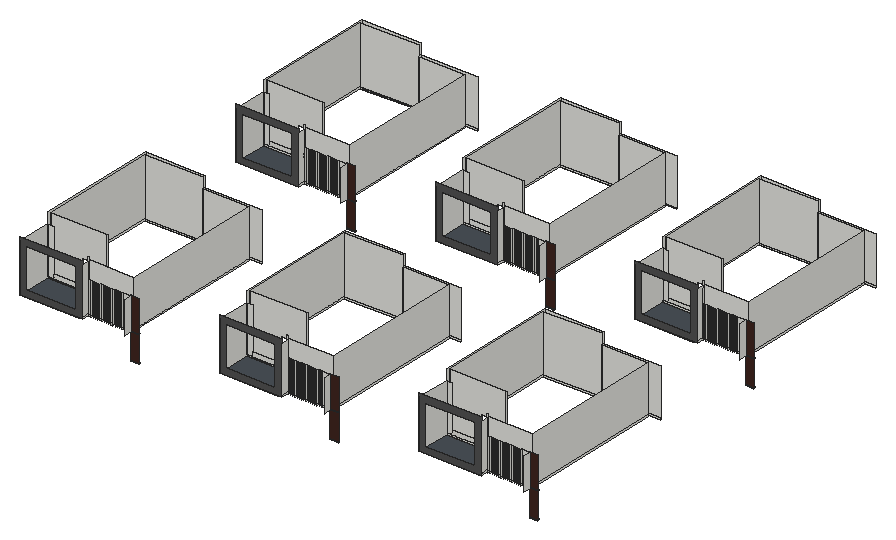
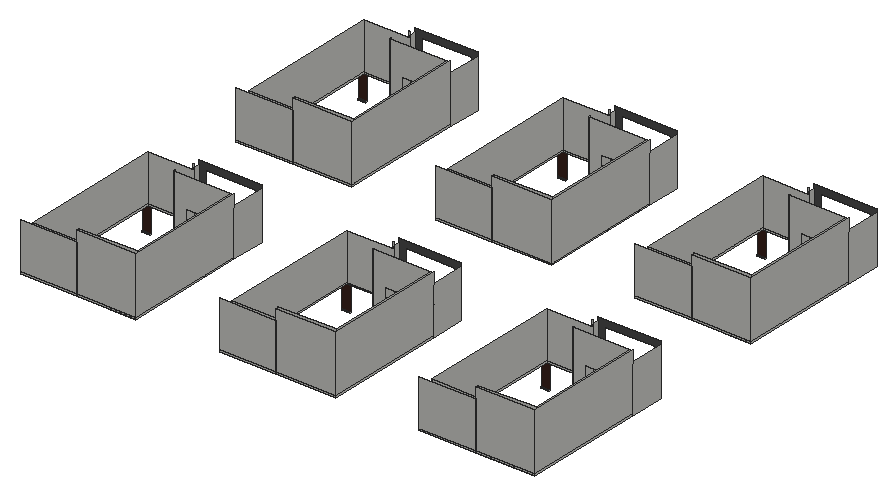
# SketchUp Ruby script. Lengths in inches.
U = 1.inch
M = Sketchup.active_model
def pt(a) = Geom::Point3d.new(a.map { |v| v * U })
def face(e, loops, mat)
  f = e.add_face(loops[0].map { |a| pt(a) })
  loops[1..].each { |l| e.add_face(l.map { |a| pt(a) }).erase! }
  f.material = f.back_material = mat if mat
  f
end
# faces: each face lists its corners as indices into pts; further lists are holes
def faces(e, pts, list, mat = nil) = list.each { |f| face(e, (f[0].is_a?(Array) ? f : [f]).map { |l| l.map { |i| pts[i] } }, mat) }
# xy, xz, yz: faces in a plane at the given z, y or x. An outline is a flat list of corners, or four numbers for a rectangle; further outlines are holes
def ring(l) = l.size == 4 ? [[l[0], l[1]], [l[2], l[1]], [l[2], l[3]], [l[0], l[3]]] : l.each_slice(2).to_a
def flat(e, list, mat, &to3) = list.each { |f| face(e, (f[0].is_a?(Array) ? f : [f]).map { |l| ring(l).map { |u, v| to3.(u, v) } }, mat) }
def xy(e, z, list, mat = nil) = flat(e, list, mat) { |x, y| [x, y, z] }
def xz(e, y, list, mat = nil) = flat(e, list, mat) { |x, z| [x, y, z] }
def yz(e, x, list, mat = nil) = flat(e, list, mat) { |y, z| [x, y, z] }
def lines(e, pts, list) = list.each { |a, b| e.add_line(pt(pts[a]), pt(pts[b])) }
# prism: a flat outline (further loops are holes) pulled along v
def prism(e, loops, v, mat = nil)
  f = face(e, loops, mat); d = Geom::Vector3d.new(v.map { |x| x * U })
  f.pushpull(f.normal.samedirection?(d) ? d.length : -d.length)
end
def box(e, o, s, mat = nil) = prism(e, [[o, [o[0] + s[0], o[1], o[2]], [o[0] + s[0], o[1] + s[1], o[2]], [o[0], o[1] + s[1], o[2]]]], [0, 0, s[2]], mat)
def at(x, y, z, deg = 0) = Geom::Transformation.translation(pt([x, y, z])) * Geom::Transformation.rotation(ORIGIN, Z_AXIS, deg.degrees)
def axes(o, x, y, z) = Geom::Transformation.new([*x, 0, *y, 0, *z, 0, *pt(o).to_a, 1])
def part(name) = M.definitions.add(name)
# library, detail: a bought-in or finely detailed component or shape, given as its bounding box
def library(name, o, s) = part(name).tap { |d| box(d.entities, o, s) }
def detail(e, o, s) = box(e.add_group.entities, o, s)
def put(e, d, t, mat = nil) = e.add_instance(d, t).tap { |i| i.material = mat if mat }
def group(e, t, mat = nil) = e.add_group.tap { |g| g.transformation = t; g.material = mat if mat }.entities
root = M.entities
M.materials.add("Glass_Tinted_Gray").color = [0, 0, 0]
M.materials["Glass_Tinted_Gray"].alpha = 0.125
M.materials.add("[0043_SaddleBrown]").color = [63, 38, 31]
M.materials.add("[0135_DarkGray]").color = [81, 81, 81]
M.materials.add("[Formica Blue]").color = [73, 80, 86]
M.materials.add("[Mirror 02]").color = [229, 229, 229]
M.materials.add("[Terrazzo Light Blue]").color = [196, 214, 227]
c1 = part("PENTEK_RP Fineline 50S_Sliding_DoorCase_E1")
box(c1.entities,[0,0,0],[1.51,3.66,99.27],"[0135_DarkGray]")
c2 = part("PENTEK_RP Fineline 50S_SlidingDooe_Case_E2")
box(c2.entities,[0,0,0],[96.25,3.66,1.51],"[0135_DarkGray]")
c3 = part("pentek_RP Fineline 50S_SlidingDoor_Case")
put(c3.entities,c1,at(97.76,0,0))
put(c3.entities,c2,at(1.51,0,0))
put(c3.entities,c1,at(0,0,0))
put(c3.entities,c2,at(1.51,0,97.76))
c4 = part("PENTEK_RP Fineline 50S_SlidingDoor_GlazingBead_2")
box(c4.entities,[0,0,0],[0.56,0.59,94.39],"[0135_DarkGray]")
c5 = part("PENTEK_RP Fineline 50S_SlidingDoor_Glass")
box(c5.entities,[0,0,0],[46.58,0.16,94.39],"Glass_Tinted_Gray")
c6 = part("PENTEK_RP Fineline 50S_SlidingDoor_GlazingBead")
box(c6.entities,[0,0,0],[45.47,0.59,0.56],"[0135_DarkGray]")
c7 = part("PENTEK_RP Fineline 50S_SlidingDoor_Leaf_E1")
xy(c7.entities,0,[[0,0,0.93,1.97],[0.93,1.57,1.49,1.97]],"[0135_DarkGray]")
xy(c7.entities,96.25,[[0,0,0.93,0,0.93,1.57,1.49,1.57,1.49,1.97,0,1.97]],"[0135_DarkGray]")
xz(c7.entities,0,[[0,0,0.93,96.25]],"[0135_DarkGray]")
xz(c7.entities,1.57,[[0.93,0,1.49,95.32],[0.93,95.32,1.49,96.25]],"[0135_DarkGray]")
xz(c7.entities,1.97,[[0,0,1.49,96.25]],"[0135_DarkGray]")
yz(c7.entities,0,[[0,0,1.97,96.25]],"[0135_DarkGray]")
yz(c7.entities,0.93,[[0,0,1.57,0.93],[0,0.93,1.57,95.32],[0,95.32,1.57,96.25]],"[0135_DarkGray]")
yz(c7.entities,1.49,[[1.57,0,1.97,95.32],[1.57,95.32,1.97,96.25]],"[0135_DarkGray]")
c8 = part("PENTEK_RP Fineline 50S_SlidingDoor_Leaf_E2")
xy(c8.entities,0,[[0,0,0,1.57,0.56,1.57,0.56,1.97,46.02,1.97,46.02,1.57,46.58,1.57,46.58,0]],"[0135_DarkGray]")
xy(c8.entities,0.93,[[0,0,46.58,1.57]],"[0135_DarkGray]")
xy(c8.entities,1.49,[[0.56,1.57,46.02,1.97]],"[0135_DarkGray]")
xz(c8.entities,0,[[0,0,46.58,0.93]],"[0135_DarkGray]")
xz(c8.entities,1.57,[[0,0,0.56,0.93],[46.02,0,46.58,0.93],[0.56,0.93,46.02,1.49]],"[0135_DarkGray]")
xz(c8.entities,1.97,[[0.56,0,46.02,1.49]],"[0135_DarkGray]")
yz(c8.entities,0,[[0,0,1.57,0.93]],"[0135_DarkGray]")
yz(c8.entities,0.56,[[1.57,0,1.97,0.93],[1.57,0.93,1.97,1.49]],"[0135_DarkGray]")
yz(c8.entities,46.02,[[1.57,0,1.97,0.93],[1.57,0.93,1.97,1.49]],"[0135_DarkGray]")
yz(c8.entities,46.58,[[0,0,1.57,0.93]],"[0135_DarkGray]")
c9 = part("PENTEK_RP Fineline S_SlidingDoor_Leaf1")
put(c9.entities,c4,at(0.93,0,0.93))
put(c9.entities,c4,at(46.96,0,0.93))
put(c9.entities,c5,at(1.49,1.42,0.93))
put(c9.entities,c6,at(1.49,0,0.93))
put(c9.entities,c5,at(1.49,0.59,0.93),"[Terrazzo Light Blue]")
put(c9.entities,c7,at(0,0,0))
put(c9.entities,c7,axes([48.44,0,0],[-1,0,0],[0,1,0],[0,0,1]))
put(c9.entities,c8,axes([0.93,0,96.25],[1,0,0],[0,1,0],[0,0,-1]))
put(c9.entities,c8,at(0.93,0,0))
put(c9.entities,c6,at(1.49,0,94.77))
c10 = part("PENTEK_RP Fineline 50S_SlidingDoor_Leaf2")
put(c10.entities,c5,at(1.49,1.42,0.93))
put(c10.entities,c6,at(1.49,0,94.77))
put(c10.entities,c4,at(46.96,0,0.93))
put(c10.entities,c5,at(1.49,0.59,0.93),"[Mirror 02]")
put(c10.entities,c4,at(0.93,0,0.93))
put(c10.entities,c7,at(0,0,0))
put(c10.entities,c7,axes([48.44,0,0],[-1,0,0],[0,1,0],[0,0,1]))
put(c10.entities,c6,at(1.49,0,0.93))
put(c10.entities,c8,axes([0.93,0,96.25],[1,0,0],[0,1,0],[0,0,-1]))
put(c10.entities,c8,at(0.93,0,0))
c11 = part("PENTEK - Slimmest Steel Sliding Door / Window\#1")
put(c11.entities,c3,at(0,-1.88,-0.09))
put(c11.entities,c9,at(1.51,-2.27,1.42))
put(c11.entities,c10,at(49.32,-0.3,1.42))
xy(root,409.48,[[517.3125,438.73,547.05,442.66],[1241.75,438.73,1271.49,442.66],[1966.1875,438.73,1995.93,442.66],[517.3125,1419.08,547.05,1423.01],[1241.75,1419.08,1271.49,1423.01],
  [1966.1875,1419.08,1995.93,1423.01]])
xy(root,412.48,[[517.3125,438.72,517.3125,442.66,547.05,442.66,547.05,438.73],[1241.75,438.72,1241.75,442.66,1271.49,442.66,1271.49,438.73],[1966.1875,438.72,1966.1875,442.66,1995.93,442.66,1995.93,438.73],[517.3125,1419.07,517.3125,1423.01,547.05,1423.01,547.05,1419.08],[1241.75,1419.07,1241.75,1423.01,1271.49,1423.01,1271.49,1419.08],
  [1966.1875,1419.07,1966.1875,1423.01,1995.93,1423.01,1995.93,1419.08]],"[0043_SaddleBrown]")
xy(root,441.5,[[258.09,535.375,309.84,598.8125],[982.53,535.375,1034.28,598.8125],[1706.96,535.375,1758.71,598.8125],[258.09,1515.73,309.84,1579.16],[982.53,1515.73,1034.28,1579.16],
  [1706.96,1515.73,1758.71,1579.16]])
xy(root,485.6875,[[183.3,535.375,231.3,598.8125],[258.09,535.375,309.84,598.8125],[907.74,535.375,955.74,598.8125],[982.53,535.375,1034.28,598.8125],[1632.17,535.375,1680.17,598.8125],
  [1706.96,535.375,1758.71,598.8125],[183.3,1515.73,231.3,1579.16],[258.09,1515.73,309.84,1579.16],[907.74,1515.73,955.74,1579.16],[982.53,1515.73,1034.28,1579.16],
  [1632.17,1515.73,1680.17,1579.16],[1706.96,1515.73,1758.71,1579.16]])
xy(root,504.25,[[348.1875,412.04,348.1875,437.1,352.41,437.1,352.41,438.72,353.97,438.72,353.97,412.04],[353.97,412.04,353.97,437.1,358.875,437.1,358.875,438.72,361.3,438.72,361.3,437.1,363.73,437.1,363.73,412.04],[1072.625,412.04,1072.625,437.1,1076.85,437.1,1076.85,438.72,1078.41,438.72,1078.41,412.04],[1078.41,412.04,1078.41,437.1,1083.3125,437.1,1083.3125,438.72,1085.74,438.72,1085.74,437.1,1088.17,437.1,1088.17,412.04],[1797.0625,412.04,1797.0625,437.1,1801.29,437.1,1801.29,438.72,1802.84,438.72,1802.84,412.04],
  [1802.84,412.04,1802.84,437.1,1807.75,437.1,1807.75,438.72,1810.18,438.72,1810.18,437.1,1812.6,437.1,1812.6,412.04],[348.1875,437.1,348.1875,447.84,353.97,447.84,353.97,438.72,352.41,438.72,352.41,437.1],[361.3,437.1,363.73,438.72],[1072.625,437.1,1072.625,447.84,1078.41,447.84,1078.41,438.72,1076.85,438.72,1076.85,437.1],[1085.74,437.1,1088.17,438.72],
  [1797.0625,437.1,1797.0625,447.84,1802.84,447.84,1802.84,438.72,1801.29,438.72,1801.29,437.1],[1810.18,437.1,1812.6,438.72],[137.5,535.375,137.5,980.35,353.97,980.35,353.97,971.23,144.84,965.96,144.84,540.48,353.97,540.48,353.97,535.375],[861.9375,535.375,861.9375,980.35,1078.41,980.35,1078.41,971.23,869.28,965.96,869.28,540.48,1078.41,540.48,1078.41,535.375],[1586.375,535.375,1586.375,980.35,1802.84,980.35,1802.84,971.23,1593.72,965.96,1593.72,540.48,1802.84,540.48,1802.84,535.375],
  [144.84,540.48,353.97,598.8125],[869.28,540.48,1078.41,598.8125],[1593.72,540.48,1802.84,598.8125],[348.1875,1392.39,348.1875,1417.45,352.41,1417.45,352.41,1419.07,353.97,1419.07,353.97,1392.39],[353.97,1392.39,353.97,1417.45,358.875,1417.45,358.875,1419.07,361.3,1419.07,361.3,1417.45,363.73,1417.45,363.73,1392.39],
  [1072.625,1392.39,1072.625,1417.45,1076.85,1417.45,1076.85,1419.07,1078.41,1419.07,1078.41,1392.39],[1078.41,1392.39,1078.41,1417.45,1083.3125,1417.45,1083.3125,1419.07,1085.74,1419.07,1085.74,1417.45,1088.17,1417.45,1088.17,1392.39],[1797.0625,1392.39,1797.0625,1417.45,1801.29,1417.45,1801.29,1419.07,1802.84,1419.07,1802.84,1392.39],[1802.84,1392.39,1802.84,1417.45,1807.75,1417.45,1807.75,1419.07,1810.18,1419.07,1810.18,1417.45,1812.6,1417.45,1812.6,1392.39],[348.1875,1417.45,348.1875,1428.19,353.97,1428.19,353.97,1419.07,352.41,1419.07,352.41,1417.45],
  [361.3,1417.45,363.73,1419.07],[1072.625,1417.45,1072.625,1428.19,1078.41,1428.19,1078.41,1419.07,1076.85,1419.07,1076.85,1417.45],[1085.74,1417.45,1088.17,1419.07],[1797.0625,1417.45,1797.0625,1428.19,1802.84,1428.19,1802.84,1419.07,1801.29,1419.07,1801.29,1417.45],[1810.18,1417.45,1812.6,1419.07],
  [137.5,1515.73,137.5,1960.7,353.97,1960.7,353.97,1951.58,144.84,1946.3125,144.84,1520.83,353.97,1520.83,353.97,1515.73],[861.9375,1515.73,861.9375,1960.7,1078.41,1960.7,1078.41,1951.58,869.28,1946.3125,869.28,1520.83,1078.41,1520.83,1078.41,1515.73],[1586.375,1515.73,1586.375,1960.7,1802.84,1960.7,1802.84,1951.58,1593.72,1946.3125,1593.72,1520.83,1802.84,1520.83,1802.84,1515.73],[144.84,1520.83,353.97,1579.16],[869.28,1520.83,1078.41,1579.16],
  [1593.72,1520.83,1802.84,1579.16]])
xy(root,504.25,[[137.5,412.04,137.5,535.375,353.97,535.375,353.97,447.84,348.1875,447.84,348.1875,412.04],[861.9375,412.04,861.9375,535.375,1078.41,535.375,1078.41,447.84,1072.625,447.84,1072.625,412.04],[1586.375,412.04,1586.375,535.375,1802.84,535.375,1802.84,447.84,1797.0625,447.84,1797.0625,412.04],[137.5,1392.39,137.5,1515.73,353.97,1515.73,353.97,1428.19,348.1875,1428.19,348.1875,1392.39],[861.9375,1392.39,861.9375,1515.73,1078.41,1515.73,1078.41,1428.19,1072.625,1428.19,1072.625,1392.39],
  [1586.375,1392.39,1586.375,1515.73,1802.84,1515.73,1802.84,1428.19,1797.0625,1428.19,1797.0625,1392.39]],"[Formica Blue]")
xy(root,505.6875,[[517.3125,438.73,547.05,442.66],[1241.75,438.73,1271.49,442.66],[1966.1875,438.73,1995.93,442.66],[517.3125,1419.08,547.05,1423.01],[1241.75,1419.08,1271.49,1423.01],
  [1966.1875,1419.08,1995.93,1423.01]])
xy(root,508.42,[[517.3125,438.72,517.3125,442.66,547.05,442.66,547.05,438.73],[1241.75,438.72,1241.75,442.66,1271.49,442.66,1271.49,438.73],[1966.1875,438.72,1966.1875,442.66,1995.93,442.66,1995.93,438.73],[517.3125,1419.07,517.3125,1423.01,547.05,1423.01,547.05,1419.08],[1241.75,1419.07,1241.75,1423.01,1271.49,1423.01,1271.49,1419.08],
  [1966.1875,1419.07,1966.1875,1423.01,1995.93,1423.01,1995.93,1419.08]])
xy(root,510.25,[[137.5,535.375,137.5,980.35,353.97,980.35,353.97,971.23,144.84,965.96,144.84,540.48,353.97,540.48,353.97,535.375],[861.9375,535.375,861.9375,980.35,1078.41,980.35,1078.41,971.23,869.28,965.96,869.28,540.48,1078.41,540.48,1078.41,535.375],[1586.375,535.375,1586.375,980.35,1802.84,980.35,1802.84,971.23,1593.72,965.96,1593.72,540.48,1802.84,540.48,1802.84,535.375],[137.5,1515.73,137.5,1960.7,353.97,1960.7,353.97,1951.58,144.84,1946.3125,144.84,1520.83,353.97,1520.83,353.97,1515.73],[861.9375,1515.73,861.9375,1960.7,1078.41,1960.7,1078.41,1951.58,869.28,1946.3125,869.28,1520.83,1078.41,1520.83,1078.41,1515.73],
  [1586.375,1515.73,1586.375,1960.7,1802.84,1960.7,1802.84,1951.58,1593.72,1946.3125,1593.72,1520.83,1802.84,1520.83,1802.84,1515.73]])
xz(root,412.04,[[[137.5,504.25,363.73,693.65],[158.83,526.75,338.6875,669.8125]],[[861.9375,504.25,1088.17,693.65],[883.27,526.75,1063.125,669.8125]],[[1586.375,504.25,1812.6,693.65],[1607.71,526.75,1787.5625,669.8125]]],"[0135_DarkGray]")
xz(root,438.72,[[361.3,504.25,363.73,693.65],[1085.74,504.25,1088.17,693.65],[1810.18,504.25,1812.6,693.65],[487.0625,510.25,517.3125,620.875],[1211.5,510.25,1241.75,620.875],
  [1935.9375,510.25,1966.1875,620.875]])
xz(root,442.66,[[517.3125,409.48,547.05,412.48],[1241.75,409.48,1271.49,412.48],[1966.1875,409.48,1995.93,412.48],[517.3125,505.6875,547.05,508.42],[1241.75,505.6875,1271.49,508.42],
  [1966.1875,505.6875,1995.93,508.42]],"[0043_SaddleBrown]")
xz(root,447.84,[[348.1875,504.25,353.97,526.75],[353.97,504.25,521.63,510.25],[1072.625,504.25,1078.41,526.75],[1078.41,504.25,1246.07,510.25],[1797.0625,504.25,1802.84,526.75],
  [1802.84,504.25,1970.51,510.25],[353.97,510.25,521.63,679.3125],[1078.41,510.25,1246.07,679.3125],[1802.84,510.25,1970.51,679.3125]])
xz(root,535.375,[[137.5,504.25,353.97,510.25],[861.9375,504.25,1078.41,510.25],[1586.375,504.25,1802.84,510.25],[137.5,510.25,158.83,679.3125],[158.83,510.25,353.97,526.75],
  [861.9375,510.25,883.27,679.3125],[883.27,510.25,1078.41,526.75],[1586.375,510.25,1607.71,679.3125],[1607.71,510.25,1802.84,526.75]])
xz(root,540.48,[[144.84,504.25,353.97,510.25],[869.28,504.25,1078.41,510.25],[1593.72,504.25,1802.84,510.25],[[144.84,510.25,353.97,718],[258.09,566.5625,309.84,610.75]],[[869.28,510.25,1078.41,718],[982.53,566.5625,1034.28,610.75]],
  [[1593.72,510.25,1802.84,718],[1706.96,566.5625,1758.71,610.75]]])
xz(root,598.8125,[[258.09,441.5,309.84,485.6875],[982.53,441.5,1034.28,485.6875],[1706.96,441.5,1758.71,485.6875]])
xz(root,971.23,[[353.97,504.25,521.63,510.25],[1078.41,504.25,1246.07,510.25],[1802.84,504.25,1970.51,510.25],[353.97,510.25,521.63,679.3125],[1078.41,510.25,1246.07,679.3125],
  [1802.84,510.25,1970.51,679.3125]])
xz(root,980.35,[[137.5,504.25,353.97,510.25],[353.97,504.25,558.625,510.25],[861.9375,504.25,1078.41,510.25],[1078.41,504.25,1283.0625,510.25],[1586.375,504.25,1802.84,510.25],
  [1802.84,504.25,2007.5,510.25],[137.5,510.25,353.97,718],[353.97,510.25,558.625,679.3125],[861.9375,510.25,1078.41,718],[1078.41,510.25,1283.0625,679.3125],
  [1586.375,510.25,1802.84,718],[1802.84,510.25,2007.5,679.3125]])
xz(root,1392.39,[[[137.5,504.25,363.73,693.65],[158.83,526.75,338.6875,669.8125]],[[861.9375,504.25,1088.17,693.65],[883.27,526.75,1063.125,669.8125]],[[1586.375,504.25,1812.6,693.65],[1607.71,526.75,1787.5625,669.8125]]],"[0135_DarkGray]")
xz(root,1419.07,[[361.3,504.25,363.73,693.65],[1085.74,504.25,1088.17,693.65],[1810.18,504.25,1812.6,693.65],[487.0625,510.25,517.3125,620.875],[1211.5,510.25,1241.75,620.875],
  [1935.9375,510.25,1966.1875,620.875]])
xz(root,1423.01,[[517.3125,409.48,547.05,412.48],[1241.75,409.48,1271.49,412.48],[1966.1875,409.48,1995.93,412.48],[517.3125,505.6875,547.05,508.42],[1241.75,505.6875,1271.49,508.42],
  [1966.1875,505.6875,1995.93,508.42]],"[0043_SaddleBrown]")
xz(root,1428.19,[[348.1875,504.25,353.97,526.75],[353.97,504.25,521.63,510.25],[1072.625,504.25,1078.41,526.75],[1078.41,504.25,1246.07,510.25],[1797.0625,504.25,1802.84,526.75],
  [1802.84,504.25,1970.51,510.25],[353.97,510.25,521.63,679.3125],[1078.41,510.25,1246.07,679.3125],[1802.84,510.25,1970.51,679.3125]])
xz(root,1515.73,[[137.5,504.25,353.97,510.25],[861.9375,504.25,1078.41,510.25],[1586.375,504.25,1802.84,510.25],[137.5,510.25,158.83,679.3125],[158.83,510.25,353.97,526.75],
  [861.9375,510.25,883.27,679.3125],[883.27,510.25,1078.41,526.75],[1586.375,510.25,1607.71,679.3125],[1607.71,510.25,1802.84,526.75]])
xz(root,1520.83,[[144.84,504.25,353.97,510.25],[869.28,504.25,1078.41,510.25],[1593.72,504.25,1802.84,510.25],[[144.84,510.25,353.97,718],[258.09,566.5625,309.84,610.75]],[[869.28,510.25,1078.41,718],[982.53,566.5625,1034.28,610.75]],
  [[1593.72,510.25,1802.84,718],[1706.96,566.5625,1758.71,610.75]]])
xz(root,1579.16,[[258.09,441.5,309.84,485.6875],[982.53,441.5,1034.28,485.6875],[1706.96,441.5,1758.71,485.6875]])
xz(root,1951.58,[[353.97,504.25,521.63,510.25],[1078.41,504.25,1246.07,510.25],[1802.84,504.25,1970.51,510.25],[353.97,510.25,521.63,679.3125],[1078.41,510.25,1246.07,679.3125],
  [1802.84,510.25,1970.51,679.3125]])
xz(root,1960.7,[[137.5,504.25,353.97,510.25],[353.97,504.25,558.625,510.25],[861.9375,504.25,1078.41,510.25],[1078.41,504.25,1283.0625,510.25],[1586.375,504.25,1802.84,510.25],
  [1802.84,504.25,2007.5,510.25],[137.5,510.25,353.97,718],[353.97,510.25,558.625,679.3125],[861.9375,510.25,1078.41,718],[1078.41,510.25,1283.0625,679.3125],
  [1586.375,510.25,1802.84,718],[1802.84,510.25,2007.5,679.3125]])
yz(root,137.5,[[412.04,504.25,535.375,679.3125],[535.375,504.25,980.35,510.25],[1392.39,504.25,1515.73,679.3125],[1515.73,504.25,1960.7,510.25],[535.375,510.25,980.35,718],
  [1515.73,510.25,1960.7,718]])
yz(root,144.84,[[540.48,504.25,965.96,510.25],[1520.83,504.25,1946.3125,510.25],[540.48,510.25,965.96,718],[1520.83,510.25,1946.3125,718]])
yz(root,258.09,[[535.375,441.5,598.8125,485.6875],[1515.73,441.5,1579.16,485.6875]])
yz(root,309.84,[[535.375,441.5,598.8125,485.6875],[1515.73,441.5,1579.16,485.6875]])
yz(root,353.97,[[447.84,504.25,535.375,526.75],[535.375,504.25,540.48,510.25],[971.23,504.25,980.35,510.25],[1428.19,504.25,1515.73,526.75],[1515.73,504.25,1520.83,510.25],
  [1951.58,504.25,1960.7,510.25],[535.375,510.25,540.48,718],[971.23,510.25,980.35,679.3125],[1515.73,510.25,1520.83,718],[1951.58,510.25,1960.7,679.3125]])
yz(root,363.73,[[412.04,504.25,437.1,510.25],[437.1,504.25,438.72,510.25],[1392.39,504.25,1417.45,510.25],[1417.45,504.25,1419.07,510.25],[412.04,510.25,437.1,679.3125],
  [437.1,510.25,438.72,679.3125],[1392.39,510.25,1417.45,679.3125],[1417.45,510.25,1419.07,679.3125]])
yz(root,367.0625,[[437.1,504.25,438.72,510.25],[1417.45,504.25,1419.07,510.25],[437.1,510.25,438.72,620.875],[1417.45,510.25,1419.07,620.875]])
yz(root,375.0625,[[437.1,504.25,438.72,510.25],[1417.45,504.25,1419.07,510.25],[437.1,510.25,438.72,620.875],[1417.45,510.25,1419.07,620.875]])
yz(root,383.0625,[[437.1,504.25,438.72,510.25],[1417.45,504.25,1419.07,510.25],[437.1,510.25,438.72,620.875],[1417.45,510.25,1419.07,620.875]])
yz(root,391.0625,[[437.1,504.25,438.72,510.25],[1417.45,504.25,1419.07,510.25],[437.1,510.25,438.72,620.875],[1417.45,510.25,1419.07,620.875]])
yz(root,399.0625,[[437.1,504.25,438.72,510.25],[1417.45,504.25,1419.07,510.25],[437.1,510.25,438.72,620.875],[1417.45,510.25,1419.07,620.875]])
yz(root,407.0625,[[437.1,504.25,438.72,510.25],[1417.45,504.25,1419.07,510.25],[437.1,510.25,438.72,620.875],[1417.45,510.25,1419.07,620.875]])
yz(root,415.0625,[[437.1,504.25,438.72,510.25],[1417.45,504.25,1419.07,510.25],[437.1,510.25,438.72,620.875],[1417.45,510.25,1419.07,620.875]])
yz(root,423.0625,[[437.1,504.25,438.72,510.25],[1417.45,504.25,1419.07,510.25],[437.1,510.25,438.72,620.875],[1417.45,510.25,1419.07,620.875]])
yz(root,431.0625,[[437.1,504.25,438.72,510.25],[1417.45,504.25,1419.07,510.25],[437.1,510.25,438.72,620.875],[1417.45,510.25,1419.07,620.875]])
yz(root,439.0625,[[437.1,504.25,438.72,510.25],[1417.45,504.25,1419.07,510.25],[437.1,510.25,438.72,620.875],[1417.45,510.25,1419.07,620.875]])
yz(root,447.0625,[[437.1,504.25,438.72,510.25],[1417.45,504.25,1419.07,510.25],[437.1,510.25,438.72,620.875],[1417.45,510.25,1419.07,620.875]])
yz(root,455.0625,[[437.1,504.25,438.72,510.25],[1417.45,504.25,1419.07,510.25],[437.1,510.25,438.72,620.875],[1417.45,510.25,1419.07,620.875]])
yz(root,463.0625,[[437.1,504.25,438.72,510.25],[1417.45,504.25,1419.07,510.25],[437.1,510.25,438.72,620.875],[1417.45,510.25,1419.07,620.875]])
yz(root,471.0625,[[437.1,504.25,438.72,510.25],[1417.45,504.25,1419.07,510.25],[437.1,510.25,438.72,620.875],[1417.45,510.25,1419.07,620.875]])
yz(root,479.0625,[[437.1,504.25,438.72,510.25],[1417.45,504.25,1419.07,510.25],[437.1,510.25,438.72,620.875],[1417.45,510.25,1419.07,620.875]])
yz(root,487.0625,[[437.1,504.25,438.72,510.25],[1417.45,504.25,1419.07,510.25],[437.1,510.25,438.72,620.875],[1417.45,510.25,1419.07,620.875]])
yz(root,517.3125,[[438.73,409.48,442.66,409.48,442.66,412.48,438.72,412.48],[1419.08,409.48,1423.01,409.48,1423.01,412.48,1419.07,412.48],[412.04,504.25,438.72,504.25,438.73,505.6875,438.72,508.42,438.72,620.875,412.04,620.875],[1392.39,504.25,1419.07,504.25,1419.08,505.6875,1419.07,508.42,1419.07,620.875,1392.39,620.875],[438.73,505.6875,442.66,505.6875,442.66,508.42,438.72,508.42],
  [1419.08,505.6875,1423.01,505.6875,1423.01,508.42,1419.07,508.42]])
yz(root,521.63,[[447.84,504.25,971.23,510.25],[1428.19,504.25,1951.58,510.25],[447.84,510.25,971.23,679.3125],[1428.19,510.25,1951.58,679.3125]])
yz(root,861.9375,[[412.04,504.25,535.375,679.3125],[535.375,504.25,980.35,510.25],[1392.39,504.25,1515.73,679.3125],[1515.73,504.25,1960.7,510.25],[535.375,510.25,980.35,718],
  [1515.73,510.25,1960.7,718]])
yz(root,869.28,[[540.48,504.25,965.96,510.25],[1520.83,504.25,1946.3125,510.25],[540.48,510.25,965.96,718],[1520.83,510.25,1946.3125,718]])
yz(root,982.53,[[535.375,441.5,598.8125,485.6875],[1515.73,441.5,1579.16,485.6875]])
yz(root,1034.28,[[535.375,441.5,598.8125,485.6875],[1515.73,441.5,1579.16,485.6875]])
yz(root,1078.41,[[447.84,504.25,535.375,526.75],[535.375,504.25,540.48,510.25],[971.23,504.25,980.35,510.25],[1428.19,504.25,1515.73,526.75],[1515.73,504.25,1520.83,510.25],
  [1951.58,504.25,1960.7,510.25],[535.375,510.25,540.48,718],[971.23,510.25,980.35,679.3125],[1515.73,510.25,1520.83,718],[1951.58,510.25,1960.7,679.3125]])
yz(root,1088.17,[[412.04,504.25,437.1,510.25],[437.1,504.25,438.72,510.25],[1392.39,504.25,1417.45,510.25],[1417.45,504.25,1419.07,510.25],[412.04,510.25,437.1,679.3125],
  [437.1,510.25,438.72,679.3125],[1392.39,510.25,1417.45,679.3125],[1417.45,510.25,1419.07,679.3125]])
yz(root,1091.5,[[437.1,504.25,438.72,510.25],[1417.45,504.25,1419.07,510.25],[437.1,510.25,438.72,620.875],[1417.45,510.25,1419.07,620.875]])
yz(root,1099.5,[[437.1,504.25,438.72,510.25],[1417.45,504.25,1419.07,510.25],[437.1,510.25,438.72,620.875],[1417.45,510.25,1419.07,620.875]])
yz(root,1107.5,[[437.1,504.25,438.72,510.25],[1417.45,504.25,1419.07,510.25],[437.1,510.25,438.72,620.875],[1417.45,510.25,1419.07,620.875]])
yz(root,1115.5,[[437.1,504.25,438.72,510.25],[1417.45,504.25,1419.07,510.25],[437.1,510.25,438.72,620.875],[1417.45,510.25,1419.07,620.875]])
yz(root,1123.5,[[437.1,504.25,438.72,510.25],[1417.45,504.25,1419.07,510.25],[437.1,510.25,438.72,620.875],[1417.45,510.25,1419.07,620.875]])
yz(root,1131.5,[[437.1,504.25,438.72,510.25],[1417.45,504.25,1419.07,510.25],[437.1,510.25,438.72,620.875],[1417.45,510.25,1419.07,620.875]])
yz(root,1139.5,[[437.1,504.25,438.72,510.25],[1417.45,504.25,1419.07,510.25],[437.1,510.25,438.72,620.875],[1417.45,510.25,1419.07,620.875]])
yz(root,1147.5,[[437.1,504.25,438.72,510.25],[1417.45,504.25,1419.07,510.25],[437.1,510.25,438.72,620.875],[1417.45,510.25,1419.07,620.875]])
yz(root,1155.5,[[437.1,504.25,438.72,510.25],[1417.45,504.25,1419.07,510.25],[437.1,510.25,438.72,620.875],[1417.45,510.25,1419.07,620.875]])
yz(root,1163.5,[[437.1,504.25,438.72,510.25],[1417.45,504.25,1419.07,510.25],[437.1,510.25,438.72,620.875],[1417.45,510.25,1419.07,620.875]])
yz(root,1171.5,[[437.1,504.25,438.72,510.25],[1417.45,504.25,1419.07,510.25],[437.1,510.25,438.72,620.875],[1417.45,510.25,1419.07,620.875]])
yz(root,1179.5,[[437.1,504.25,438.72,510.25],[1417.45,504.25,1419.07,510.25],[437.1,510.25,438.72,620.875],[1417.45,510.25,1419.07,620.875]])
yz(root,1187.5,[[437.1,504.25,438.72,510.25],[1417.45,504.25,1419.07,510.25],[437.1,510.25,438.72,620.875],[1417.45,510.25,1419.07,620.875]])
yz(root,1195.5,[[437.1,504.25,438.72,510.25],[1417.45,504.25,1419.07,510.25],[437.1,510.25,438.72,620.875],[1417.45,510.25,1419.07,620.875]])
yz(root,1203.5,[[437.1,504.25,438.72,510.25],[1417.45,504.25,1419.07,510.25],[437.1,510.25,438.72,620.875],[1417.45,510.25,1419.07,620.875]])
yz(root,1211.5,[[437.1,504.25,438.72,510.25],[1417.45,504.25,1419.07,510.25],[437.1,510.25,438.72,620.875],[1417.45,510.25,1419.07,620.875]])
yz(root,1241.75,[[438.73,409.48,442.66,409.48,442.66,412.48,438.72,412.48],[1419.08,409.48,1423.01,409.48,1423.01,412.48,1419.07,412.48],[412.04,504.25,438.72,504.25,438.73,505.6875,438.72,508.42,438.72,620.875,412.04,620.875],[1392.39,504.25,1419.07,504.25,1419.08,505.6875,1419.07,508.42,1419.07,620.875,1392.39,620.875],[438.73,505.6875,442.66,505.6875,442.66,508.42,438.72,508.42],
  [1419.08,505.6875,1423.01,505.6875,1423.01,508.42,1419.07,508.42]])
yz(root,1246.07,[[447.84,504.25,971.23,510.25],[1428.19,504.25,1951.58,510.25],[447.84,510.25,971.23,679.3125],[1428.19,510.25,1951.58,679.3125]])
yz(root,1586.375,[[412.04,504.25,535.375,679.3125],[535.375,504.25,980.35,510.25],[1392.39,504.25,1515.73,679.3125],[1515.73,504.25,1960.7,510.25],[535.375,510.25,980.35,718],
  [1515.73,510.25,1960.7,718]])
yz(root,1593.72,[[540.48,504.25,965.96,510.25],[1520.83,504.25,1946.3125,510.25],[540.48,510.25,965.96,718],[1520.83,510.25,1946.3125,718]])
yz(root,1706.96,[[535.375,441.5,598.8125,485.6875],[1515.73,441.5,1579.16,485.6875]])
yz(root,1758.71,[[535.375,441.5,598.8125,485.6875],[1515.73,441.5,1579.16,485.6875]])
yz(root,1802.84,[[447.84,504.25,535.375,526.75],[535.375,504.25,540.48,510.25],[971.23,504.25,980.35,510.25],[1428.19,504.25,1515.73,526.75],[1515.73,504.25,1520.83,510.25],
  [1951.58,504.25,1960.7,510.25],[535.375,510.25,540.48,718],[971.23,510.25,980.35,679.3125],[1515.73,510.25,1520.83,718],[1951.58,510.25,1960.7,679.3125]])
yz(root,1812.6,[[412.04,504.25,437.1,510.25],[437.1,504.25,438.72,510.25],[1392.39,504.25,1417.45,510.25],[1417.45,504.25,1419.07,510.25],[412.04,510.25,437.1,679.3125],
  [437.1,510.25,438.72,679.3125],[1392.39,510.25,1417.45,679.3125],[1417.45,510.25,1419.07,679.3125]])
yz(root,1815.9375,[[437.1,504.25,438.72,510.25],[1417.45,504.25,1419.07,510.25],[437.1,510.25,438.72,620.875],[1417.45,510.25,1419.07,620.875]])
yz(root,1823.9375,[[437.1,504.25,438.72,510.25],[1417.45,504.25,1419.07,510.25],[437.1,510.25,438.72,620.875],[1417.45,510.25,1419.07,620.875]])
yz(root,1831.9375,[[437.1,504.25,438.72,510.25],[1417.45,504.25,1419.07,510.25],[437.1,510.25,438.72,620.875],[1417.45,510.25,1419.07,620.875]])
yz(root,1839.9375,[[437.1,504.25,438.72,510.25],[1417.45,504.25,1419.07,510.25],[437.1,510.25,438.72,620.875],[1417.45,510.25,1419.07,620.875]])
yz(root,1847.9375,[[437.1,504.25,438.72,510.25],[1417.45,504.25,1419.07,510.25],[437.1,510.25,438.72,620.875],[1417.45,510.25,1419.07,620.875]])
yz(root,1855.9375,[[437.1,504.25,438.72,510.25],[1417.45,504.25,1419.07,510.25],[437.1,510.25,438.72,620.875],[1417.45,510.25,1419.07,620.875]])
yz(root,1863.9375,[[437.1,504.25,438.72,510.25],[1417.45,504.25,1419.07,510.25],[437.1,510.25,438.72,620.875],[1417.45,510.25,1419.07,620.875]])
yz(root,1871.9375,[[437.1,504.25,438.72,510.25],[1417.45,504.25,1419.07,510.25],[437.1,510.25,438.72,620.875],[1417.45,510.25,1419.07,620.875]])
yz(root,1879.9375,[[437.1,504.25,438.72,510.25],[1417.45,504.25,1419.07,510.25],[437.1,510.25,438.72,620.875],[1417.45,510.25,1419.07,620.875]])
yz(root,1887.9375,[[437.1,504.25,438.72,510.25],[1417.45,504.25,1419.07,510.25],[437.1,510.25,438.72,620.875],[1417.45,510.25,1419.07,620.875]])
yz(root,1895.9375,[[437.1,504.25,438.72,510.25],[1417.45,504.25,1419.07,510.25],[437.1,510.25,438.72,620.875],[1417.45,510.25,1419.07,620.875]])
yz(root,1903.9375,[[437.1,504.25,438.72,510.25],[1417.45,504.25,1419.07,510.25],[437.1,510.25,438.72,620.875],[1417.45,510.25,1419.07,620.875]])
yz(root,1911.9375,[[437.1,504.25,438.72,510.25],[1417.45,504.25,1419.07,510.25],[437.1,510.25,438.72,620.875],[1417.45,510.25,1419.07,620.875]])
yz(root,1919.9375,[[437.1,504.25,438.72,510.25],[1417.45,504.25,1419.07,510.25],[437.1,510.25,438.72,620.875],[1417.45,510.25,1419.07,620.875]])
yz(root,1927.9375,[[437.1,504.25,438.72,510.25],[1417.45,504.25,1419.07,510.25],[437.1,510.25,438.72,620.875],[1417.45,510.25,1419.07,620.875]])
yz(root,1935.9375,[[437.1,504.25,438.72,510.25],[1417.45,504.25,1419.07,510.25],[437.1,510.25,438.72,620.875],[1417.45,510.25,1419.07,620.875]])
yz(root,1966.1875,[[438.73,409.48,442.66,409.48,442.66,412.48,438.72,412.48],[1419.08,409.48,1423.01,409.48,1423.01,412.48,1419.07,412.48],[412.04,504.25,438.72,504.25,438.73,505.6875,438.72,508.42,438.72,620.875,412.04,620.875],[1392.39,504.25,1419.07,504.25,1419.08,505.6875,1419.07,508.42,1419.07,620.875,1392.39,620.875],[438.73,505.6875,442.66,505.6875,442.66,508.42,438.72,508.42],
  [1419.08,505.6875,1423.01,505.6875,1423.01,508.42,1419.07,508.42]])
yz(root,1970.51,[[447.84,504.25,971.23,510.25],[1428.19,504.25,1951.58,510.25],[447.84,510.25,971.23,679.3125],[1428.19,510.25,1951.58,679.3125]])
p = [[547.05,438.73,412.48],[547.05,438.73,505.6875],[517.3125,438.73,505.6875],[517.3125,438.72,504.25],[517.3125,438.72,412.48],[1271.49,438.73,412.48],
  [1271.49,438.73,505.6875],[1241.75,438.73,505.6875],[1241.75,438.72,504.25],[1241.75,438.72,412.48],[1995.93,438.73,412.48],[1995.93,438.73,505.6875],
  [1966.1875,438.73,505.6875],[1966.1875,438.72,504.25],[1966.1875,438.72,412.48],[547.05,1419.08,412.48],[547.05,1419.08,505.6875],[517.3125,1419.08,505.6875],
  [517.3125,1419.07,504.25],[517.3125,1419.07,412.48],[1271.49,1419.08,412.48],[1271.49,1419.08,505.6875],[1241.75,1419.08,505.6875],[1241.75,1419.07,504.25],
  [1241.75,1419.07,412.48],[1995.93,1419.08,412.48],[1995.93,1419.08,505.6875],[1966.1875,1419.08,505.6875],[1966.1875,1419.07,504.25],[1966.1875,1419.07,412.48],
  [487.0625,438.72,504.25],[487.0625,438.72,510.25],[517.3125,438.72,510.25],[517.3125,438.72,508.42],[1211.5,438.72,504.25],[1211.5,438.72,510.25],
  [1241.75,438.72,510.25],[1241.75,438.72,508.42],[1935.9375,438.72,504.25],[1935.9375,438.72,510.25],[1966.1875,438.72,510.25],[1966.1875,438.72,508.42],
  [144.84,965.96,504.25],[353.97,971.23,504.25],[353.97,971.23,510.25],[144.84,965.96,510.25],[869.28,965.96,504.25],[1078.41,971.23,504.25],
  [1078.41,971.23,510.25],[869.28,965.96,510.25],[1593.72,965.96,504.25],[1802.84,971.23,504.25],[1802.84,971.23,510.25],[1593.72,965.96,510.25],
  [487.0625,1419.07,504.25],[487.0625,1419.07,510.25],[517.3125,1419.07,510.25],[517.3125,1419.07,508.42],[1211.5,1419.07,504.25],[1211.5,1419.07,510.25],
  [1241.75,1419.07,510.25],[1241.75,1419.07,508.42],[1935.9375,1419.07,504.25],[1935.9375,1419.07,510.25],[1966.1875,1419.07,510.25],[1966.1875,1419.07,508.42],
  [144.84,1946.3125,504.25],[353.97,1951.58,504.25],[353.97,1951.58,510.25],[144.84,1946.3125,510.25],[869.28,1946.3125,504.25],[1078.41,1951.58,504.25],
  [1078.41,1951.58,510.25],[869.28,1946.3125,510.25],[1593.72,1946.3125,504.25],[1802.84,1951.58,504.25],[1802.84,1951.58,510.25],[1593.72,1946.3125,510.25],
  [547.05,438.73,508.42],[547.05,438.73,623.5625],[517.3125,438.73,623.5625],[517.3125,438.72,620.875],[1271.49,438.73,508.42],[1271.49,438.73,623.5625],
  [1241.75,438.73,623.5625],[1241.75,438.72,620.875],[1995.93,438.73,508.42],[1995.93,438.73,623.5625],[1966.1875,438.73,623.5625],[1966.1875,438.72,620.875],
  [547.05,1419.08,508.42],[547.05,1419.08,623.5625],[517.3125,1419.08,623.5625],[517.3125,1419.07,620.875],[1271.49,1419.08,508.42],[1271.49,1419.08,623.5625],
  [1241.75,1419.08,623.5625],[1241.75,1419.07,620.875],[1995.93,1419.08,508.42],[1995.93,1419.08,623.5625],[1966.1875,1419.08,623.5625],[1966.1875,1419.07,620.875],
  [353.97,971.23,679.3125],[353.97,971.23,718],[144.84,965.96,718],[1078.41,971.23,679.3125],[1078.41,971.23,718],[869.28,965.96,718],
  [1802.84,971.23,679.3125],[1802.84,971.23,718],[1593.72,965.96,718],[353.97,1951.58,679.3125],[353.97,1951.58,718],[144.84,1946.3125,718],
  [1078.41,1951.58,679.3125],[1078.41,1951.58,718],[869.28,1946.3125,718],[1802.84,1951.58,679.3125],[1802.84,1951.58,718],[1593.72,1946.3125,718],
  [1078.41,447.84,510.25],[1078.41,438.72,510.25],[1802.84,447.84,510.25],[1802.84,438.72,510.25],[353.97,447.84,510.25],[353.97,438.72,510.25],
  [1078.41,1428.19,510.25],[1078.41,1419.07,510.25],[1802.84,1428.19,510.25],[1802.84,1419.07,510.25],[353.97,1428.19,510.25],[353.97,1419.07,510.25]]
faces(root,p,[[0,1,2,3,4],[5,6,7,8,9],[10,11,12,13,14],[15,16,17,18,19],[20,21,22,23,24],[25,26,27,28,29],[78,79,80,81,32,33],[82,83,84,85,36,37],
  [86,87,88,89,40,41],[90,91,92,93,56,57],[94,95,96,97,60,61],[98,99,100,101,64,65]],"[0043_SaddleBrown]")
faces(root,p,[[3,30,31,32,33,2],[8,34,35,36,37,7],[13,38,39,40,41,12],[42,43,44,45],[46,47,48,49],[50,51,52,53],[18,54,55,56,57,17],[23,58,59,60,61,22],
  [28,62,63,64,65,27],[66,67,68,69],[70,71,72,73],[74,75,76,77],[45,44,102,103,104],[49,48,105,106,107],[53,52,108,109,110],[69,68,111,112,113],
  [73,72,114,115,116],[77,76,117,118,119]])
lines(root,p,[[120,121],[122,123],[124,125],[126,127],[128,129],[130,131]])
put(root,c11,axes([258.09,1515.73,441.5],[0.52129,0,0],[0,0.44,0],[0,0,0.44603]))
put(root,c11,axes([982.53,1515.73,441.5],[0.52129,0,0],[0,0.44,0],[0,0,0.44603]))
put(root,c11,axes([1706.96,1515.73,441.5],[0.52129,0,0],[0,0.44,0],[0,0,0.44603]))
put(root,c11,axes([982.53,535.375,441.5],[0.52129,0,0],[0,0.44,0],[0,0,0.44603]))
put(root,c11,axes([1706.96,535.375,441.5],[0.52129,0,0],[0,0.44,0],[0,0,0.44603]))
put(root,c11,axes([258.09,535.375,441.5],[0.52129,0,0],[0,0.44,0],[0,0,0.44603]))
